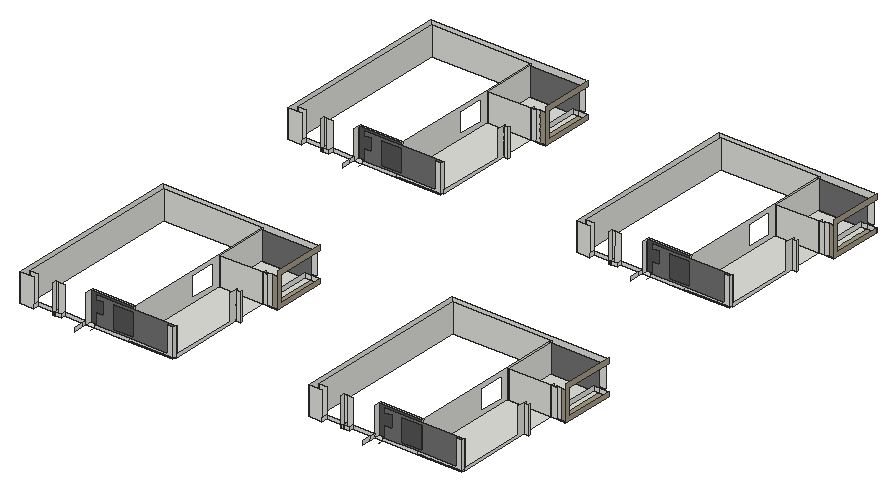
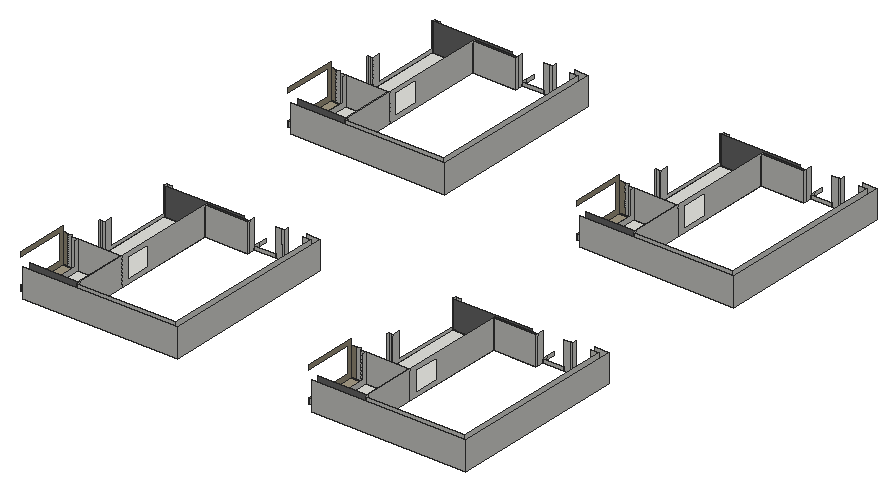
# SketchUp Ruby script. Lengths in inches.
U = 1.inch
M = Sketchup.active_model
def pt(a) = Geom::Point3d.new(a.map { |v| v * U })
def face(e, loops, mat)
  f = e.add_face(loops[0].map { |a| pt(a) })
  loops[1..].each { |l| e.add_face(l.map { |a| pt(a) }).erase! }
  f.material = f.back_material = mat if mat
  f
end
# faces: each face lists its corners as indices into pts; further lists are holes
def faces(e, pts, list, mat = nil) = list.each { |f| face(e, (f[0].is_a?(Array) ? f : [f]).map { |l| l.map { |i| pts[i] } }, mat) }
# xy, xz, yz: faces in a plane at the given z, y or x. An outline is a flat list of corners, or four numbers for a rectangle; further outlines are holes
def ring(l) = l.size == 4 ? [[l[0], l[1]], [l[2], l[1]], [l[2], l[3]], [l[0], l[3]]] : l.each_slice(2).to_a
def flat(e, list, mat, &to3) = list.each { |f| face(e, (f[0].is_a?(Array) ? f : [f]).map { |l| ring(l).map { |u, v| to3.(u, v) } }, mat) }
def xy(e, z, list, mat = nil) = flat(e, list, mat) { |x, y| [x, y, z] }
def xz(e, y, list, mat = nil) = flat(e, list, mat) { |x, z| [x, y, z] }
def yz(e, x, list, mat = nil) = flat(e, list, mat) { |y, z| [x, y, z] }
def lines(e, pts, list) = list.each { |a, b| e.add_line(pt(pts[a]), pt(pts[b])) }
# prism: a flat outline (further loops are holes) pulled along v
def prism(e, loops, v, mat = nil)
  f = face(e, loops, mat); d = Geom::Vector3d.new(v.map { |x| x * U })
  f.pushpull(f.normal.samedirection?(d) ? d.length : -d.length)
end
def box(e, o, s, mat = nil) = prism(e, [[o, [o[0] + s[0], o[1], o[2]], [o[0] + s[0], o[1] + s[1], o[2]], [o[0], o[1] + s[1], o[2]]]], [0, 0, s[2]], mat)
def at(x, y, z, deg = 0) = Geom::Transformation.translation(pt([x, y, z])) * Geom::Transformation.rotation(ORIGIN, Z_AXIS, deg.degrees)
def axes(o, x, y, z) = Geom::Transformation.new([*x, 0, *y, 0, *z, 0, *pt(o).to_a, 1])
def part(name) = M.definitions.add(name)
# library, detail: a bought-in or finely detailed component or shape, given as its bounding box
def library(name, o, s) = part(name).tap { |d| box(d.entities, o, s) }
def detail(e, o, s) = box(e.add_group.entities, o, s)
def put(e, d, t, mat = nil) = e.add_instance(d, t).tap { |i| i.material = mat if mat }
def group(e, t, mat = nil) = e.add_group.tap { |g| g.transformation = t; g.material = mat if mat }.entities
root = M.entities
M.materials.add("[Color M05]").color = [114, 114, 114]
M.materials.add("[Color M06]").color = [86, 86, 86]
M.materials.add("[Concrete Tile]").color = [165, 155, 133]
M.materials.add("[Granite Brown]").color = [89, 59, 61]
xy(root,1140,[[523.04,1822.9375,557.4,1846],[653.67,1822.9375,704.25,1835.1875],[1741.23,1822.9375,1775.59,1846],[1871.86,1822.9375,1922.4375,1835.1875],[557.4,1835.1875,704.25,1846],
  [704.25,1835.1875,890.875,2295.875],[1775.59,1835.1875,1922.4375,1846],[1922.4375,1835.1875,2109.0625,2295.875],[523.04,1846,557.4,1856.375],[557.4,1846,704.25,1856.375],
  [1741.23,1846,1775.59,1856.375],[1775.59,1846,1922.4375,1856.375],[894.3125,2148.83,913.875,2156.01],[2112.5,2148.83,2132.0625,2156.01],[704.25,2295.875,710.125,2518.89],
  [710.125,2295.875,890.875,2518.89],[890.875,2295.875,913.875,2518.89],[1922.4375,2295.875,1928.3125,2518.89],[1928.3125,2295.875,2109.0625,2518.89],[2109.0625,2295.875,2132.0625,2518.89],
  [704.25,2518.89,890.875,2531.375],[1922.4375,2518.89,2109.0625,2531.375],[523.04,3237.625,557.4,3260.6875],[653.67,3237.625,704.25,3249.875],[1741.23,3237.625,1775.59,3260.6875],
  [1871.86,3237.625,1922.4375,3249.875],[557.4,3249.875,704.25,3260.6875],[704.25,3249.875,890.875,3710.5625],[1775.59,3249.875,1922.4375,3260.6875],[1922.4375,3249.875,2109.0625,3710.5625],
  [523.04,3260.6875,557.4,3271.0625],[557.4,3260.6875,704.25,3271.0625],[1741.23,3260.6875,1775.59,3271.0625],[1775.59,3260.6875,1922.4375,3271.0625],[894.3125,3563.51,913.875,3570.7],
  [2112.5,3563.51,2132.0625,3570.7],[704.25,3710.5625,710.125,3933.57],[710.125,3710.5625,890.875,3933.57],[890.875,3710.5625,913.875,3933.57],[1922.4375,3710.5625,1928.3125,3933.57],
  [1928.3125,3710.5625,2109.0625,3933.57],[2109.0625,3710.5625,2132.0625,3933.57],[704.25,3933.57,890.875,3946.0625],[1922.4375,3933.57,2109.0625,3946.0625]])
xy(root,1140,[[913.875,2295.875,954.6875,2518.89],[2132.0625,2295.875,2172.875,2518.89],[913.875,3710.5625,954.6875,3933.57],[2132.0625,3710.5625,2172.875,3933.57]],"[Concrete Tile]")
xy(root,1140,[[557.4,1822.9375,557.88,1835.1875],[1775.59,1822.9375,1776.07,1835.1875],[557.4,3237.625,557.88,3249.875],[1775.59,3237.625,1776.07,3249.875]],"[Granite Brown]")
xy(root,1142,[[704.25,1822.9375,890.875,1835.1875],[1922.4375,1822.9375,2109.0625,1835.1875],[704.25,3237.625,890.875,3249.875],[1922.4375,3237.625,2109.0625,3249.875]])
xz(root,1799.9375,[[262.875,1140,319.53,1260],[1481.0625,1140,1537.72,1260]])
xz(root,1806.5625,[[404.32,1140,404.32,1155.4375,393.59,1155.49,393.51,1140.05],[404.32,1140,404.4,1155.4375,404.32,1155.4375],[404.32,1140,431.33,1140,431.33,1155.4375,404.4,1155.4375],[1622.51,1140,1622.51,1155.4375,1611.78,1155.49,1611.7,1140.05],[1622.51,1140,1622.59,1155.4375,1622.51,1155.4375],
  [1622.51,1140,1649.52,1140,1649.52,1155.4375,1622.59,1155.4375]])
xz(root,1822.9375,[[285.875,1140,319.53,1260],[319.53,1140,404.32,1140,393.51,1140.05,393.59,1155.4375,319.53,1155.4375],[404.32,1140,393.51,1140.05,393.59,1155.4375,404.32,1155.4375],[404.32,1140,404.92,1260,394.11,1260,393.59,1155.4375,404.32,1155.4375],[404.32,1140,404.92,1260,431.33,1260,431.33,1140],
  [431.33,1140,523.04,1155.4375],[557.88,1140,704.25,1152.6875],[704.25,1140,890.875,1142],[1504.0625,1140,1537.72,1260],[1537.72,1140,1622.51,1140,1611.7,1140.05,1611.78,1155.4375,1537.72,1155.4375],
  [1622.51,1140,1611.7,1140.05,1611.78,1155.4375,1622.51,1155.4375],[1622.51,1140,1623.11,1260,1612.3,1260,1611.78,1155.4375,1622.51,1155.4375],[1622.51,1140,1623.11,1260,1649.52,1260,1649.52,1140],[1649.52,1140,1741.23,1155.4375],[1776.07,1140,1922.4375,1152.6875],
  [1922.4375,1140,2109.0625,1142],[704.25,1142,704.25,1152.6875,869.48,1152.6875,869.48,1260,890.875,1260,890.875,1142],[1922.4375,1142,1922.4375,1152.6875,2087.67,1152.6875,2087.67,1260,2109.0625,1260,2109.0625,1142]])
xz(root,1835.1875,[[704.25,1140,890.875,1142],[890.875,1140,894.3125,1260],[1922.4375,1140,2109.0625,1142],[2109.0625,1140,2112.5,1260]])
xz(root,1835.1875,[[[557.88,1140,704.25,1140,704.25,1142,890.875,1142,890.875,1260,557.88,1260,557.88,1242.26,588.66,1242.26,588.66,1189.98,557.88,1189.98],[646.53,1150.95,646.53,1151.26,625.7,1151.26,625.7,1249.08,715.63,1249.08,715.63,1150.95]],[[1776.07,1140,1922.4375,1140,1922.4375,1142,2109.0625,1142,2109.0625,1260,1776.07,1260,1776.07,1242.26,1806.84,1242.26,1806.84,1189.98,1776.07,1189.98],[1864.72,1150.95,1864.72,1151.26,1843.88,1151.26,1843.88,1249.08,1933.82,1249.08,1933.82,1150.95]]],"[Color M05]")
xz(root,1846,[[523.04,1140,704.25,1260],[1741.23,1140,1922.4375,1260]],"[Color M06]")
xz(root,1856.375,[[523.04,1140,704.25,1260],[1741.23,1140,1922.4375,1260]])
xz(root,2148.83,[[894.3125,1140,913.875,1260],[2112.5,1140,2132.0625,1260]])
xz(root,2156.01,[[894.3125,1140,913.875,1157.36],[2112.5,1140,2132.0625,1157.36]])
xz(root,2295.875,[[704.25,1140,710.125,1260],[710.125,1140,890.875,1260],[890.875,1140,913.875,1260],[913.875,1140,930.75,1141.75],[930.75,1140,954.6875,1141.75],
  [1922.4375,1140,1928.3125,1260],[1928.3125,1140,2109.0625,1260],[2109.0625,1140,2132.0625,1260],[2132.0625,1140,2148.9375,1141.75],[2148.9375,1140,2172.875,1141.75],
  [913.875,1141.75,930.75,1266],[2132.0625,1141.75,2148.9375,1266]])
xz(root,2295.875,[[930.75,1141.75,954.6875,1266],[2148.9375,1141.75,2172.875,1266]],"[Concrete Tile]")
xz(root,2518.89,[[704.25,1140,710.125,1260],[890.875,1140,913.875,1160.8125],[913.875,1140,954.6875,1160.8125],[1922.4375,1140,1928.3125,1260],[2109.0625,1140,2132.0625,1160.8125],
  [2132.0625,1140,2172.875,1160.8125]])
xz(root,2518.89,[[710.125,1140,890.875,1140,890.875,1160.8125,913.875,1160.8125,913.875,1260,710.125,1260],[1928.3125,1140,2109.0625,1140,2109.0625,1160.8125,2132.0625,1160.8125,2132.0625,1260,1928.3125,1260]],"[Color M05]")
xz(root,2531.375,[[285.875,1140,704.25,1260],[1504.0625,1140,1922.4375,1260]])
xz(root,2554.375,[[262.875,1140,913.875,1260],[1481.0625,1140,2132.0625,1260]])
xz(root,3214.625,[[262.875,1140,319.53,1260],[1481.0625,1140,1537.72,1260]])
xz(root,3221.25,[[404.32,1140,404.32,1155.4375,393.59,1155.49,393.51,1140.05],[404.32,1140,404.4,1155.4375,404.32,1155.4375],[404.32,1140,431.33,1140,431.33,1155.4375,404.4,1155.4375],[1622.51,1140,1622.51,1155.4375,1611.78,1155.49,1611.7,1140.05],[1622.51,1140,1622.59,1155.4375,1622.51,1155.4375],
  [1622.51,1140,1649.52,1140,1649.52,1155.4375,1622.59,1155.4375]])
xz(root,3237.625,[[285.875,1140,319.53,1260],[319.53,1140,404.32,1140,393.51,1140.05,393.59,1155.4375,319.53,1155.4375],[404.32,1140,393.51,1140.05,393.59,1155.4375,404.32,1155.4375],[404.32,1140,404.92,1260,394.11,1260,393.59,1155.4375,404.32,1155.4375],[404.32,1140,404.92,1260,431.33,1260,431.33,1140],
  [431.33,1140,523.04,1155.4375],[557.88,1140,704.25,1152.6875],[704.25,1140,890.875,1142],[1504.0625,1140,1537.72,1260],[1537.72,1140,1622.51,1140,1611.7,1140.05,1611.78,1155.4375,1537.72,1155.4375],
  [1622.51,1140,1611.7,1140.05,1611.78,1155.4375,1622.51,1155.4375],[1622.51,1140,1623.11,1260,1612.3,1260,1611.78,1155.4375,1622.51,1155.4375],[1622.51,1140,1623.11,1260,1649.52,1260,1649.52,1140],[1649.52,1140,1741.23,1155.4375],[1776.07,1140,1922.4375,1152.6875],
  [1922.4375,1140,2109.0625,1142],[704.25,1142,704.25,1152.6875,869.48,1152.6875,869.48,1260,890.875,1260,890.875,1142],[1922.4375,1142,1922.4375,1152.6875,2087.67,1152.6875,2087.67,1260,2109.0625,1260,2109.0625,1142]])
xz(root,3249.875,[[704.25,1140,890.875,1142],[890.875,1140,894.3125,1260],[1922.4375,1140,2109.0625,1142],[2109.0625,1140,2112.5,1260]])
xz(root,3249.875,[[[557.88,1140,704.25,1140,704.25,1142,890.875,1142,890.875,1260,557.88,1260,557.88,1242.26,588.66,1242.26,588.66,1189.98,557.88,1189.98],[646.53,1150.95,646.53,1151.26,625.7,1151.26,625.7,1249.08,715.63,1249.08,715.63,1150.95]],[[1776.07,1140,1922.4375,1140,1922.4375,1142,2109.0625,1142,2109.0625,1260,1776.07,1260,1776.07,1242.26,1806.84,1242.26,1806.84,1189.98,1776.07,1189.98],[1864.72,1150.95,1864.72,1151.26,1843.88,1151.26,1843.88,1249.08,1933.82,1249.08,1933.82,1150.95]]],"[Color M05]")
xz(root,3260.6875,[[523.04,1140,704.25,1260],[1741.23,1140,1922.4375,1260]],"[Color M06]")
xz(root,3271.0625,[[523.04,1140,704.25,1260],[1741.23,1140,1922.4375,1260]])
xz(root,3563.51,[[894.3125,1140,913.875,1260],[2112.5,1140,2132.0625,1260]])
xz(root,3570.7,[[894.3125,1140,913.875,1157.36],[2112.5,1140,2132.0625,1157.36]])
xz(root,3710.5625,[[704.25,1140,710.125,1260],[710.125,1140,890.875,1260],[890.875,1140,913.875,1260],[913.875,1140,930.75,1141.75],[930.75,1140,954.6875,1141.75],
  [1922.4375,1140,1928.3125,1260],[1928.3125,1140,2109.0625,1260],[2109.0625,1140,2132.0625,1260],[2132.0625,1140,2148.9375,1141.75],[2148.9375,1140,2172.875,1141.75],
  [913.875,1141.75,930.75,1266],[2132.0625,1141.75,2148.9375,1266]])
xz(root,3710.5625,[[930.75,1141.75,954.6875,1266],[2148.9375,1141.75,2172.875,1266]],"[Concrete Tile]")
xz(root,3933.57,[[704.25,1140,710.125,1260],[890.875,1140,913.875,1160.8125],[913.875,1140,954.6875,1160.8125],[1922.4375,1140,1928.3125,1260],[2109.0625,1140,2132.0625,1160.8125],
  [2132.0625,1140,2172.875,1160.8125]])
xz(root,3933.57,[[710.125,1140,890.875,1140,890.875,1160.8125,913.875,1160.8125,913.875,1260,710.125,1260],[1928.3125,1140,2109.0625,1140,2109.0625,1160.8125,2132.0625,1160.8125,2132.0625,1260,1928.3125,1260]],"[Color M05]")
xz(root,3946.0625,[[285.875,1140,704.25,1260],[1504.0625,1140,1922.4375,1260]])
xz(root,3969.0625,[[262.875,1140,913.875,1260],[1481.0625,1140,2132.0625,1260]])
yz(root,262.875,[[1799.9375,1140,2554.375,1260],[3214.625,1140,3969.0625,1260]])
yz(root,285.875,[[1822.9375,1140,2531.375,1260],[3237.625,1140,3946.0625,1260]])
yz(root,319.53,[[1799.9375,1140,1822.9375,1155.4375],[3214.625,1140,3237.625,1155.4375]])
yz(root,404.32,[[1806.5625,1140,1822.9375,1155.4375],[3221.25,1140,3237.625,1155.4375]])
yz(root,431.33,[[1806.5625,1140,1822.9375,1155.4375],[3221.25,1140,3237.625,1155.4375]])
yz(root,523.04,[[1763.25,1140,1799.9375,1155.4375],[1799.9375,1140,1822.9375,1155.4375],[1822.9375,1140,1846,1260],[1846,1140,1856.375,1260],[3177.9375,1140,3214.625,1155.4375],
  [3214.625,1140,3237.625,1155.4375],[3237.625,1140,3260.6875,1260],[3260.6875,1140,3271.0625,1260]])
yz(root,704.25,[[1822.9375,1140,1835.1875,1142],[1846,1140,1856.375,1260],[[1856.375,1140,2295.875,1260],[2156.01,1157.36,2266.33,1243.04]],[2295.875,1140,2518.89,1260],[2518.89,1140,2531.375,1260],
  [3237.625,1140,3249.875,1142],[3260.6875,1140,3271.0625,1260],[[3271.0625,1140,3710.5625,1260],[3570.7,1157.36,3681.01,1243.04]],[3710.5625,1140,3933.57,1260],[3933.57,1140,3946.0625,1260]])
yz(root,710.125,[[2295.875,1140,2518.89,1260],[3710.5625,1140,3933.57,1260]])
yz(root,890.875,[[1822.9375,1140,1835.1875,1142],[2295.875,1140,2295.875,1260,2310.68,1260,2310.68,1160.8125,2518.89,1160.8125,2518.89,1140],[3237.625,1140,3249.875,1142],[3710.5625,1140,3710.5625,1260,3725.37,1260,3725.37,1160.8125,3933.57,1160.8125,3933.57,1140],[1822.9375,1142,1835.1875,1260],
  [3237.625,1142,3249.875,1260]])
yz(root,894.3125,[[1835.1875,1140,2148.83,1140,2148.83,1260,2117.96,1260,2117.96,1152.6875,1835.1875,1152.6875],[2148.83,1140,2156.01,1260],[3249.875,1140,3563.51,1140,3563.51,1260,3532.65,1260,3532.65,1152.6875,3249.875,1152.6875],[3563.51,1140,3570.7,1260]])
yz(root,913.875,[[2148.83,1140,2156.01,1260],[3563.51,1140,3570.7,1260]])
yz(root,954.6875,[[2295.875,1140,2518.89,1140,2518.89,1160.8125,2310.68,1160.8125,2310.68,1266,2518.89,1266,2518.89,1286.8125,2295.875,1286.8125],[3710.5625,1140,3933.57,1140,3933.57,1160.8125,3725.37,1160.8125,3725.37,1266,3933.57,1266,3933.57,1286.8125,3710.5625,1286.8125]],"[Concrete Tile]")
yz(root,1481.0625,[[1799.9375,1140,2554.375,1260],[3214.625,1140,3969.0625,1260]])
yz(root,1504.0625,[[1822.9375,1140,2531.375,1260],[3237.625,1140,3946.0625,1260]])
yz(root,1537.72,[[1799.9375,1140,1822.9375,1155.4375],[3214.625,1140,3237.625,1155.4375]])
yz(root,1622.51,[[1806.5625,1140,1822.9375,1155.4375],[3221.25,1140,3237.625,1155.4375]])
yz(root,1649.52,[[1806.5625,1140,1822.9375,1155.4375],[3221.25,1140,3237.625,1155.4375]])
yz(root,1741.23,[[1763.25,1140,1799.9375,1155.4375],[1799.9375,1140,1822.9375,1155.4375],[1822.9375,1140,1846,1260],[1846,1140,1856.375,1260],[3177.9375,1140,3214.625,1155.4375],
  [3214.625,1140,3237.625,1155.4375],[3237.625,1140,3260.6875,1260],[3260.6875,1140,3271.0625,1260]])
yz(root,1922.4375,[[1822.9375,1140,1835.1875,1142],[1846,1140,1856.375,1260],[[1856.375,1140,2295.875,1260],[2156.01,1157.36,2266.33,1243.04]],[2295.875,1140,2518.89,1260],[2518.89,1140,2531.375,1260],
  [3237.625,1140,3249.875,1142],[3260.6875,1140,3271.0625,1260],[[3271.0625,1140,3710.5625,1260],[3570.7,1157.36,3681.01,1243.04]],[3710.5625,1140,3933.57,1260],[3933.57,1140,3946.0625,1260]])
yz(root,1928.3125,[[2295.875,1140,2518.89,1260],[3710.5625,1140,3933.57,1260]])
yz(root,2109.0625,[[1822.9375,1140,1835.1875,1142],[2295.875,1140,2295.875,1260,2310.68,1260,2310.68,1160.8125,2518.89,1160.8125,2518.89,1140],[3237.625,1140,3249.875,1142],[3710.5625,1140,3710.5625,1260,3725.37,1260,3725.37,1160.8125,3933.57,1160.8125,3933.57,1140],[1822.9375,1142,1835.1875,1260],
  [3237.625,1142,3249.875,1260]])
yz(root,2112.5,[[1835.1875,1140,2148.83,1140,2148.83,1260,2117.96,1260,2117.96,1152.6875,1835.1875,1152.6875],[2148.83,1140,2156.01,1260],[3249.875,1140,3563.51,1140,3563.51,1260,3532.65,1260,3532.65,1152.6875,3249.875,1152.6875],[3563.51,1140,3570.7,1260]])
yz(root,2132.0625,[[2148.83,1140,2156.01,1260],[3563.51,1140,3570.7,1260]])
yz(root,2172.875,[[2295.875,1140,2518.89,1140,2518.89,1160.8125,2310.68,1160.8125,2310.68,1266,2518.89,1266,2518.89,1286.8125,2295.875,1286.8125],[3710.5625,1140,3933.57,1140,3933.57,1160.8125,3725.37,1160.8125,3725.37,1266,3933.57,1266,3933.57,1286.8125,3710.5625,1286.8125]],"[Concrete Tile]")
p = [[404.32,1822.9375,1140],[404.32,1806.5625,1140],[393.51,1806.5625,1140.05],[393.51,1822.9375,1140.05],[1622.51,1822.9375,1140],[1622.51,1806.5625,1140],
  [1611.7,1806.5625,1140.05],[1611.7,1822.9375,1140.05],[404.32,3237.625,1140],[404.32,3221.25,1140],[393.51,3221.25,1140.05],[393.51,3237.625,1140.05],
  [1622.51,3237.625,1140],[1622.51,3221.25,1140],[1611.7,3221.25,1140.05],[1611.7,3237.625,1140.05],[393.59,1806.5625,1155.49],[394.11,1806.5625,1260.05],
  [394.11,1822.9375,1260.05],[394.11,1822.9375,1260],[393.59,1822.9375,1155.4375],[1611.78,1806.5625,1155.49],[1612.3,1806.5625,1260.05],[1612.3,1822.9375,1260.05],
  [1612.3,1822.9375,1260],[1611.78,1822.9375,1155.4375],[393.59,3221.25,1155.49],[394.11,3221.25,1260.05],[394.11,3237.625,1260.05],[394.11,3237.625,1260],
  [393.59,3237.625,1155.4375],[1611.78,3221.25,1155.49],[1612.3,3221.25,1260.05],[1612.3,3237.625,1260.05],[1612.3,3237.625,1260],[1611.78,3237.625,1155.4375],
  [1775.59,1799.9375,1140],[1775.59,1822.9375,1140],[557.4,1799.9375,1140],[557.4,1822.9375,1140],[1775.59,3214.625,1140],[1775.59,3237.625,1140],
  [557.4,3214.625,1140],[557.4,3237.625,1140]]
faces(root,p,[[0,1,2,3],[4,5,6,7],[8,9,10,11],[12,13,14,15],[3,2,16,17,18,19,20],[7,6,21,22,23,24,25],[11,10,26,27,28,29,30],[15,14,31,32,33,34,35]])
lines(root,p,[[36,37],[38,39],[40,41],[42,43]])
